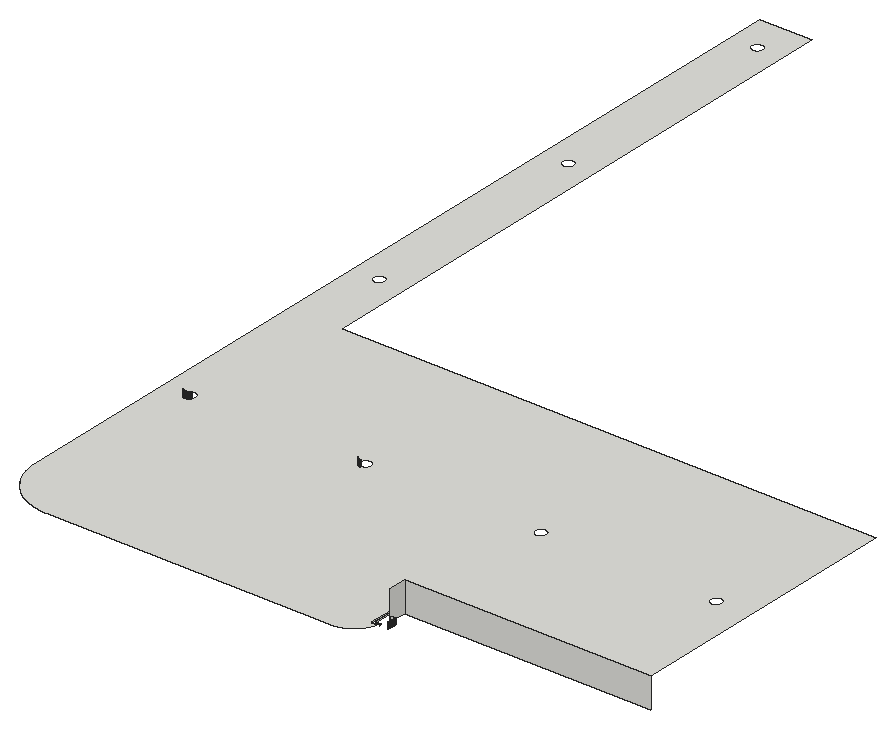
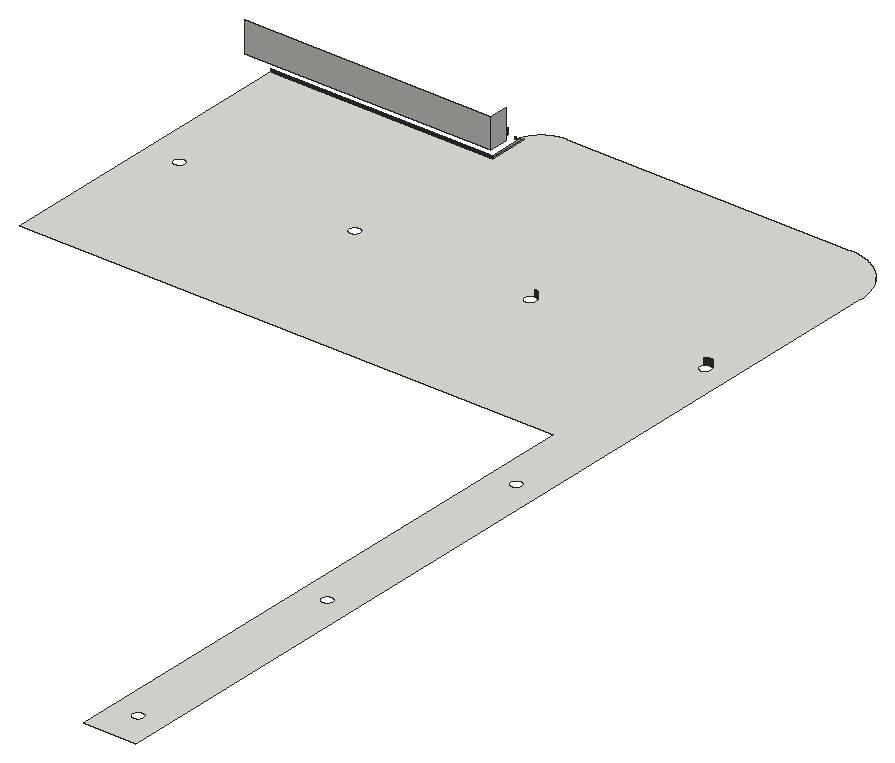
# SketchUp Ruby script. Lengths in inches.
U = 1.inch
M = Sketchup.active_model
def pt(a) = Geom::Point3d.new(a.map { |v| v * U })
def face(e, loops, mat)
  f = e.add_face(loops[0].map { |a| pt(a) })
  loops[1..].each { |l| e.add_face(l.map { |a| pt(a) }).erase! }
  f.material = f.back_material = mat if mat
  f
end
# faces: each face lists its corners as indices into pts; further lists are holes
def faces(e, pts, list, mat = nil) = list.each { |f| face(e, (f[0].is_a?(Array) ? f : [f]).map { |l| l.map { |i| pts[i] } }, mat) }
# xy, xz, yz: faces in a plane at the given z, y or x. An outline is a flat list of corners, or four numbers for a rectangle; further outlines are holes
def ring(l) = l.size == 4 ? [[l[0], l[1]], [l[2], l[1]], [l[2], l[3]], [l[0], l[3]]] : l.each_slice(2).to_a
def flat(e, list, mat, &to3) = list.each { |f| face(e, (f[0].is_a?(Array) ? f : [f]).map { |l| ring(l).map { |u, v| to3.(u, v) } }, mat) }
def xy(e, z, list, mat = nil) = flat(e, list, mat) { |x, y| [x, y, z] }
def xz(e, y, list, mat = nil) = flat(e, list, mat) { |x, z| [x, y, z] }
def yz(e, x, list, mat = nil) = flat(e, list, mat) { |y, z| [x, y, z] }
def lines(e, pts, list) = list.each { |a, b| e.add_line(pt(pts[a]), pt(pts[b])) }
# prism: a flat outline (further loops are holes) pulled along v
def prism(e, loops, v, mat = nil)
  f = face(e, loops, mat); d = Geom::Vector3d.new(v.map { |x| x * U })
  f.pushpull(f.normal.samedirection?(d) ? d.length : -d.length)
end
def box(e, o, s, mat = nil) = prism(e, [[o, [o[0] + s[0], o[1], o[2]], [o[0] + s[0], o[1] + s[1], o[2]], [o[0], o[1] + s[1], o[2]]]], [0, 0, s[2]], mat)
def at(x, y, z, deg = 0) = Geom::Transformation.translation(pt([x, y, z])) * Geom::Transformation.rotation(ORIGIN, Z_AXIS, deg.degrees)
def axes(o, x, y, z) = Geom::Transformation.new([*x, 0, *y, 0, *z, 0, *pt(o).to_a, 1])
def part(name) = M.definitions.add(name)
# library, detail: a bought-in or finely detailed component or shape, given as its bounding box
def library(name, o, s) = part(name).tap { |d| box(d.entities, o, s) }
def detail(e, o, s) = box(e.add_group.entities, o, s)
def put(e, d, t, mat = nil) = e.add_instance(d, t).tap { |i| i.material = mat if mat }
def group(e, t, mat = nil) = e.add_group.tap { |g| g.transformation = t; g.material = mat if mat }.entities
root = M.entities
M.materials.add("1496 AP 8293 CARBON COPY").color = [58, 58, 58]
xy(root,258,[[[43.63,69,43.27,69.01,42.9,69.02,42.53,69.04,42.17,69.06,41.8,69.09,41.4375,69.12,41.07,69.15,40.71,69.19,40.35,69.24,39.98,69.29,39.62,69.34,39.26,69.4,38.18,69.61,37.46,69.77,37.11,69.86,36.75,69.95,36.05,70.15,35.35,70.37,34.65,70.61,34.31,70.73,33.97,70.86,33.625,70.99,33.28,71.13,32.95,71.27,32.61,71.42,32.28,71.57,31.29,72.05,30.96,72.22,30.64,72.39,30,72.75,29.68,72.9375,29.37,73.125,29.06,73.32,28.44,73.72,28.14,73.92,27.84,74.13,27.54,74.35,27.25,74.56,26.95,74.79,26.67,75.01,26.38,75.24,26.1,75.47,25.26,76.19,24.99,76.4375,24.73,76.69,24.46,76.94,23.94,77.46,23.69,77.73,23.4375,77.99,23.19,78.26,22.47,79.1,22.24,79.38,22.01,79.67,21.79,79.95,21.56,80.25,21.35,80.54,21.13,80.84,20.92,81.14,20.72,81.44,20.32,82.06,20.125,82.37,19.9375,82.68,19.75,83,19.39,83.64,19.22,83.96,19.05,84.29,18.57,85.28,18.42,85.61,18.27,85.95,18.13,86.28,17.99,86.625,17.86,86.97,17.73,87.31,17.61,87.65,17.37,88.35,17.15,89.05,16.95,89.75,16.86,90.11,16.77,90.46,16.61,91.18,16.4,92.26,16.34,92.62,16.29,92.98,16.24,93.35,16.19,93.71,16.15,94.07,16.12,94.4375,16.09,94.8,16.06,95.17,16.04,95.53,16.02,95.9,16.01,96.27,16,96.63,16,550,42,550,42,256,309,256,309,99,198,99,198,80,200.2,80,200.15,79.86,200.01,79.46,199.9375,79.27,199.86,79.07,199.78,78.88,199.7,78.68,199.62,78.49,199.35,77.92,199.26,77.74,199.16,77.55,199.0625,77.37,198.96,77.18,198.86,77,198.53,76.46,198.42,76.29,198.3,76.11,198.1875,75.9375,198.07,75.77,197.94,75.6,197.82,75.43,197.56,75.09,197.17,74.61,196.89,74.29,196.61,73.99,196.46,73.84,196.3125,73.6875,196.16,73.54,196.01,73.39,195.71,73.11,195.39,72.83,194.91,72.44,194.57,72.18,194.4,72.06,194.23,71.93,194.0625,71.8125,193.89,71.7,193.71,71.58,193.54,71.47,193,71.14,192.82,71.04,192.63,70.9375,192.45,70.84,192.26,70.74,192.08,70.65,191.51,70.38,191.32,70.3,191.12,70.22,190.93,70.14,190.73,70.0625,190.54,69.99,189.94,69.78,189.34,69.6,189.14,69.55,188.9375,69.49,188.74,69.44,188.53,69.39,188.33,69.35,188.12,69.31,187.92,69.27,187.71,69.23,187.5,69.2,187.3,69.17,186.88,69.11,186.46,69.07,186.26,69.05,186.05,69.03,185.63,69.01,185.42,69.01,185.21,69],[28.92,410.83,29.08,410.83,29.16,410.84,29.24,410.84,29.3125,410.85,29.39,410.86,29.55,410.88,29.7,410.92,29.78,410.9375,29.85,410.96,29.93,410.98,30,411.01,30.08,411.03,30.15,411.0625,30.22,411.09,30.36,411.16,30.57,411.28,30.63,411.32,30.7,411.36,30.76,411.41,30.83,411.45,31.01,411.6,31.18,411.77,31.23,411.83,31.28,411.88,31.33,411.95,31.43,412.07,31.47,412.13,31.52,412.2,31.56,412.27,31.6,412.33,31.64,412.4,31.67,412.47,31.71,412.54,31.74,412.61,31.77,412.69,31.83,412.83,31.85,412.91,31.875,412.98,31.9,413.06,31.92,413.13,31.93,413.21,31.95,413.29,31.96,413.36,32,413.68,32,413.99,31.98,414.15,31.97,414.22,31.95,414.38,31.93,414.46,31.92,414.53,31.9,414.61,31.875,414.69,31.85,414.76,31.83,414.83,31.8,414.91,31.74,415.05,31.71,415.125,31.67,415.2,31.64,415.26,31.52,415.47,31.47,415.53,31.43,415.6,31.18,415.9,31.12,415.95,31.07,416.01,31.01,416.0625,30.95,416.11,30.83,416.21,30.76,416.26,30.7,416.31,30.63,416.35,30.57,416.39,30.36,416.51,30.08,416.63,30,416.66,29.93,416.6875,29.85,416.71,29.78,416.73,29.7,416.75,29.625,416.77,29.55,416.78,29.47,416.8,29.39,416.81,29.3125,416.82,29.24,416.82,29.16,416.83,28.84,416.83,28.76,416.82,28.6875,416.82,28.61,416.81,28.53,416.8,28.45,416.78,28.375,416.77,28.3,416.75,28.22,416.73,28.15,416.71,28.07,416.6875,28,416.66,27.92,416.63,27.64,416.51,27.43,416.39,27.37,416.35,27.3,416.31,27.24,416.26,27.17,416.21,27.05,416.11,26.99,416.0625,26.93,416.01,26.88,415.95,26.82,415.9,26.57,415.6,26.53,415.53,26.48,415.47,26.36,415.26,26.33,415.2,26.29,415.125,26.26,415.05,26.2,414.91,26.17,414.83,26.15,414.76,26.125,414.69,26.1,414.61,26.08,414.53,26.07,414.46,26.05,414.38,26.03,414.22,26.02,414.15,26,413.99,26,413.68,26.04,413.36,26.05,413.29,26.07,413.21,26.08,413.13,26.1,413.06,26.125,412.98,26.15,412.91,26.17,412.83,26.23,412.69,26.26,412.61,26.29,412.54,26.33,412.47,26.36,412.4,26.4,412.33,26.44,412.27,26.48,412.2,26.53,412.13,26.57,412.07,26.67,411.95,26.72,411.88,26.77,411.83,26.82,411.77,26.99,411.6,27.17,411.45,27.24,411.41,27.3,411.36,27.37,411.32,27.43,411.28,27.64,411.16,27.78,411.09,27.85,411.0625,27.92,411.03,28,411.01,28.07,410.98,28.15,410.96,28.22,410.9375,28.3,410.92,28.45,410.88,28.61,410.86,28.6875,410.85,28.76,410.84,28.84,410.84],[28.84,292.67,29.16,292.67,29.24,292.68,29.3125,292.68,29.39,292.69,29.47,292.7,29.55,292.72,29.625,292.73,29.7,292.75,29.78,292.77,29.85,292.79,29.93,292.8125,30,292.84,30.08,292.87,30.36,292.99,30.57,293.11,30.63,293.15,30.7,293.19,30.76,293.24,30.83,293.29,30.95,293.39,31.01,293.4375,31.07,293.49,31.12,293.55,31.18,293.6,31.43,293.9,31.47,293.97,31.52,294.03,31.64,294.24,31.67,294.3,31.71,294.375,31.74,294.45,31.8,294.59,31.83,294.67,31.85,294.74,31.875,294.81,31.9,294.89,31.92,294.97,31.93,295.04,31.95,295.12,31.97,295.28,31.98,295.35,32,295.51,32,295.82,31.96,296.14,31.95,296.21,31.93,296.29,31.92,296.37,31.9,296.44,31.875,296.52,31.85,296.59,31.83,296.67,31.77,296.81,31.74,296.89,31.71,296.96,31.67,297.03,31.64,297.1,31.6,297.17,31.56,297.23,31.52,297.3,31.47,297.37,31.43,297.43,31.33,297.55,31.28,297.62,31.23,297.67,31.18,297.73,31.01,297.9,30.83,298.05,30.76,298.09,30.7,298.14,30.63,298.18,30.57,298.22,30.36,298.34,30.22,298.41,30.15,298.4375,30.08,298.47,30,298.49,29.93,298.52,29.85,298.54,29.78,298.5625,29.7,298.58,29.55,298.62,29.39,298.64,29.3125,298.65,29.24,298.66,29.16,298.66,29.08,298.67,28.92,298.67,28.84,298.66,28.76,298.66,28.6875,298.65,28.61,298.64,28.45,298.62,28.3,298.58,28.22,298.5625,28.15,298.54,28.07,298.52,28,298.49,27.92,298.47,27.85,298.4375,27.78,298.41,27.64,298.34,27.43,298.22,27.37,298.18,27.3,298.14,27.24,298.09,27.17,298.05,26.99,297.9,26.82,297.73,26.77,297.67,26.72,297.62,26.67,297.55,26.57,297.43,26.53,297.37,26.48,297.3,26.44,297.23,26.4,297.17,26.36,297.1,26.33,297.03,26.29,296.96,26.26,296.89,26.23,296.81,26.17,296.67,26.15,296.59,26.125,296.52,26.1,296.44,26.08,296.37,26.07,296.29,26.05,296.21,26.04,296.14,26,295.82,26,295.51,26.02,295.35,26.03,295.28,26.05,295.12,26.07,295.04,26.08,294.97,26.1,294.89,26.125,294.81,26.15,294.74,26.17,294.67,26.2,294.59,26.26,294.45,26.29,294.375,26.33,294.3,26.36,294.24,26.48,294.03,26.53,293.97,26.57,293.9,26.82,293.6,26.88,293.55,26.93,293.49,26.99,293.4375,27.05,293.39,27.17,293.29,27.24,293.24,27.3,293.19,27.37,293.15,27.43,293.11,27.64,292.99,27.92,292.87,28,292.84,28.07,292.8125,28.15,292.79,28.22,292.77,28.3,292.75,28.375,292.73,28.45,292.72,28.53,292.7,28.61,292.69,28.6875,292.68,28.76,292.68],[28.84,174.5,29.16,174.5,29.24,174.51,29.3125,174.52,29.39,174.53,29.55,174.55,29.625,174.57,29.7,174.58,29.78,174.6,29.85,174.625,29.93,174.65,30,174.67,30.08,174.7,30.29,174.79,30.36,174.83,30.43,174.86,30.57,174.94,30.63,174.98,30.7,175.03,30.76,175.07,30.83,175.12,31.07,175.32,31.12,175.38,31.18,175.43,31.38,175.67,31.43,175.74,31.47,175.8,31.52,175.87,31.56,175.93,31.64,176.07,31.67,176.14,31.71,176.21,31.8,176.42,31.83,176.5,31.85,176.57,31.875,176.65,31.9,176.72,31.92,176.8,31.93,176.875,31.95,176.95,31.97,177.11,31.98,177.1875,31.99,177.26,32,177.34,32,177.66,31.99,177.74,31.98,177.8125,31.97,177.89,31.95,178.05,31.93,178.125,31.92,178.2,31.9,178.28,31.875,178.35,31.85,178.43,31.83,178.5,31.8,178.58,31.71,178.79,31.67,178.86,31.64,178.93,31.56,179.07,31.52,179.13,31.47,179.2,31.43,179.26,31.38,179.33,31.18,179.57,31.12,179.62,31.07,179.68,30.83,179.88,30.76,179.93,30.7,179.97,30.63,180.02,30.57,180.06,30.43,180.14,30.36,180.17,30.29,180.21,30.08,180.3,30,180.33,29.93,180.35,29.85,180.375,29.78,180.4,29.7,180.42,29.625,180.43,29.55,180.45,29.39,180.47,29.3125,180.48,29.24,180.49,29.16,180.5,28.84,180.5,28.76,180.49,28.6875,180.48,28.61,180.47,28.45,180.45,28.375,180.43,28.3,180.42,28.22,180.4,28.15,180.375,28.07,180.35,28,180.33,27.92,180.3,27.71,180.21,27.64,180.17,27.57,180.14,27.43,180.06,27.37,180.02,27.3,179.97,27.24,179.93,27.17,179.88,26.93,179.68,26.88,179.62,26.82,179.57,26.62,179.33,26.57,179.26,26.53,179.2,26.48,179.13,26.44,179.07,26.36,178.93,26.33,178.86,26.29,178.79,26.2,178.58,26.17,178.5,26.15,178.43,26.125,178.35,26.1,178.28,26.08,178.2,26.07,178.125,26.05,178.05,26.03,177.89,26.02,177.8125,26.01,177.74,26,177.66,26,177.34,26.01,177.26,26.02,177.1875,26.03,177.11,26.05,176.95,26.07,176.875,26.08,176.8,26.1,176.72,26.125,176.65,26.15,176.57,26.17,176.5,26.2,176.42,26.29,176.21,26.33,176.14,26.36,176.07,26.44,175.93,26.48,175.87,26.53,175.8,26.57,175.74,26.62,175.67,26.82,175.43,26.88,175.38,26.93,175.32,27.17,175.12,27.24,175.07,27.3,175.03,27.37,174.98,27.43,174.94,27.57,174.86,27.64,174.83,27.71,174.79,27.92,174.7,28,174.67,28.07,174.65,28.15,174.625,28.22,174.6,28.3,174.58,28.375,174.57,28.45,174.55,28.61,174.53,28.6875,174.52,28.76,174.51],[28.84,529,29.16,529,29.24,529.01,29.3125,529.02,29.39,529.03,29.55,529.05,29.625,529.07,29.7,529.08,29.78,529.1,29.85,529.125,29.93,529.15,30,529.17,30.08,529.2,30.29,529.29,30.36,529.33,30.43,529.36,30.57,529.44,30.63,529.48,30.7,529.53,30.76,529.57,30.83,529.62,31.07,529.82,31.12,529.88,31.18,529.93,31.38,530.17,31.43,530.24,31.47,530.3,31.52,530.37,31.56,530.43,31.64,530.57,31.67,530.64,31.71,530.71,31.8,530.92,31.83,531,31.85,531.07,31.875,531.15,31.9,531.22,31.92,531.3,31.93,531.375,31.95,531.45,31.97,531.61,31.98,531.6875,31.99,531.76,32,531.84,32,532.16,31.99,532.24,31.98,532.3125,31.97,532.39,31.95,532.55,31.93,532.625,31.92,532.7,31.9,532.78,31.875,532.85,31.85,532.93,31.83,533,31.8,533.08,31.71,533.29,31.67,533.36,31.64,533.43,31.56,533.57,31.52,533.63,31.47,533.7,31.43,533.76,31.38,533.83,31.18,534.07,31.12,534.12,31.07,534.18,30.83,534.38,30.76,534.43,30.7,534.47,30.63,534.52,30.57,534.56,30.43,534.64,30.36,534.67,30.29,534.71,30.08,534.8,30,534.83,29.93,534.85,29.85,534.875,29.78,534.9,29.7,534.92,29.625,534.93,29.55,534.95,29.39,534.97,29.3125,534.98,29.24,534.99,29.16,535,28.84,535,28.76,534.99,28.6875,534.98,28.61,534.97,28.45,534.95,28.375,534.93,28.3,534.92,28.22,534.9,28.15,534.875,28.07,534.85,28,534.83,27.92,534.8,27.71,534.71,27.64,534.67,27.57,534.64,27.43,534.56,27.37,534.52,27.3,534.47,27.24,534.43,27.17,534.38,26.93,534.18,26.88,534.12,26.82,534.07,26.62,533.83,26.57,533.76,26.53,533.7,26.48,533.63,26.44,533.57,26.36,533.43,26.33,533.36,26.29,533.29,26.2,533.08,26.17,533,26.15,532.93,26.125,532.85,26.1,532.78,26.08,532.7,26.07,532.625,26.05,532.55,26.03,532.39,26.02,532.3125,26.01,532.24,26,532.16,26,531.84,26.01,531.76,26.02,531.6875,26.03,531.61,26.05,531.45,26.07,531.375,26.08,531.3,26.1,531.22,26.125,531.15,26.15,531.07,26.17,531,26.2,530.92,26.29,530.71,26.33,530.64,26.36,530.57,26.44,530.43,26.48,530.37,26.53,530.3,26.57,530.24,26.62,530.17,26.82,529.93,26.88,529.88,26.93,529.82,27.17,529.62,27.24,529.57,27.3,529.53,27.37,529.48,27.43,529.44,27.57,529.36,27.64,529.33,27.71,529.29,27.92,529.2,28,529.17,28.07,529.15,28.15,529.125,28.22,529.1,28.3,529.08,28.375,529.07,28.45,529.05,28.61,529.03,28.6875,529.02,28.76,529.01],[116.51,174.5,116.82,174.5,117.14,174.54,117.21,174.55,117.29,174.57,117.37,174.58,117.44,174.6,117.52,174.625,117.59,174.65,117.67,174.67,117.81,174.73,117.89,174.76,117.96,174.79,118.03,174.83,118.1,174.86,118.17,174.9,118.23,174.94,118.3,174.98,118.37,175.03,118.43,175.07,118.55,175.17,118.62,175.22,118.67,175.27,118.73,175.32,118.9,175.49,119.05,175.67,119.09,175.74,119.14,175.8,119.18,175.87,119.22,175.93,119.34,176.14,119.41,176.28,119.4375,176.35,119.47,176.42,119.49,176.5,119.52,176.57,119.54,176.65,119.5625,176.72,119.58,176.8,119.62,176.95,119.64,177.11,119.65,177.1875,119.66,177.26,119.66,177.34,119.67,177.42,119.67,177.58,119.66,177.66,119.66,177.74,119.65,177.8125,119.64,177.89,119.62,178.05,119.58,178.2,119.5625,178.28,119.54,178.35,119.52,178.43,119.49,178.5,119.47,178.58,119.4375,178.65,119.41,178.72,119.34,178.86,119.22,179.07,119.18,179.13,119.14,179.2,119.09,179.26,119.05,179.33,118.9,179.51,118.73,179.68,118.67,179.73,118.62,179.78,118.55,179.83,118.43,179.93,118.37,179.97,118.3,180.02,118.23,180.06,118.17,180.1,118.1,180.14,118.03,180.17,117.96,180.21,117.89,180.24,117.81,180.27,117.67,180.33,117.59,180.35,117.52,180.375,117.44,180.4,117.37,180.42,117.29,180.43,117.21,180.45,117.14,180.46,116.82,180.5,116.51,180.5,116.35,180.48,116.28,180.47,116.12,180.45,116.04,180.43,115.97,180.42,115.89,180.4,115.81,180.375,115.74,180.35,115.67,180.33,115.59,180.3,115.45,180.24,115.375,180.21,115.3,180.17,115.24,180.14,115.03,180.02,114.97,179.97,114.9,179.93,114.6,179.68,114.55,179.62,114.49,179.57,114.4375,179.51,114.39,179.45,114.29,179.33,114.24,179.26,114.19,179.2,114.15,179.13,114.11,179.07,113.99,178.86,113.87,178.58,113.84,178.5,113.8125,178.43,113.79,178.35,113.77,178.28,113.75,178.2,113.73,178.125,113.72,178.05,113.7,177.97,113.69,177.89,113.68,177.8125,113.68,177.74,113.67,177.66,113.67,177.34,113.68,177.26,113.68,177.1875,113.69,177.11,113.7,177.03,113.72,176.95,113.73,176.875,113.75,176.8,113.77,176.72,113.79,176.65,113.8125,176.57,113.84,176.5,113.87,176.42,113.99,176.14,114.11,175.93,114.15,175.87,114.19,175.8,114.24,175.74,114.29,175.67,114.39,175.55,114.4375,175.49,114.49,175.43,114.55,175.38,114.6,175.32,114.9,175.07,114.97,175.03,115.03,174.98,115.24,174.86,115.3,174.83,115.375,174.79,115.45,174.76,115.59,174.7,115.67,174.67,115.74,174.65,115.81,174.625,115.89,174.6,115.97,174.58,116.04,174.57,116.12,174.55,116.28,174.53,116.35,174.52],[204.18,174.5,204.49,174.5,204.65,174.52,204.72,174.53,204.88,174.55,204.96,174.57,205.03,174.58,205.11,174.6,205.19,174.625,205.26,174.65,205.33,174.67,205.41,174.7,205.55,174.76,205.625,174.79,205.7,174.83,205.76,174.86,205.97,174.98,206.03,175.03,206.1,175.07,206.4,175.32,206.45,175.38,206.51,175.43,206.5625,175.49,206.61,175.55,206.71,175.67,206.76,175.74,206.81,175.8,206.85,175.87,206.89,175.93,207.01,176.14,207.13,176.42,207.16,176.5,207.1875,176.57,207.21,176.65,207.23,176.72,207.25,176.8,207.27,176.875,207.28,176.95,207.3,177.03,207.31,177.11,207.32,177.1875,207.32,177.26,207.33,177.34,207.33,177.66,207.32,177.74,207.32,177.8125,207.31,177.89,207.3,177.97,207.28,178.05,207.27,178.125,207.25,178.2,207.23,178.28,207.21,178.35,207.1875,178.43,207.16,178.5,207.13,178.58,207.01,178.86,206.89,179.07,206.85,179.13,206.81,179.2,206.76,179.26,206.71,179.33,206.61,179.45,206.5625,179.51,206.51,179.57,206.45,179.62,206.4,179.68,206.1,179.93,206.03,179.97,205.97,180.02,205.76,180.14,205.7,180.17,205.625,180.21,205.55,180.24,205.41,180.3,205.33,180.33,205.26,180.35,205.19,180.375,205.11,180.4,205.03,180.42,204.96,180.43,204.88,180.45,204.72,180.47,204.65,180.48,204.49,180.5,204.18,180.5,203.86,180.46,203.79,180.45,203.71,180.43,203.63,180.42,203.56,180.4,203.48,180.375,203.41,180.35,203.33,180.33,203.19,180.27,203.11,180.24,203.04,180.21,202.97,180.17,202.9,180.14,202.83,180.1,202.77,180.06,202.7,180.02,202.63,179.97,202.57,179.93,202.45,179.83,202.38,179.78,202.33,179.73,202.27,179.68,202.1,179.51,201.95,179.33,201.91,179.26,201.86,179.2,201.82,179.13,201.78,179.07,201.66,178.86,201.59,178.72,201.5625,178.65,201.53,178.58,201.51,178.5,201.48,178.43,201.46,178.35,201.4375,178.28,201.42,178.2,201.38,178.05,201.36,177.89,201.35,177.8125,201.34,177.74,201.34,177.66,201.33,177.58,201.33,177.42,201.34,177.34,201.34,177.26,201.35,177.1875,201.36,177.11,201.38,176.95,201.42,176.8,201.4375,176.72,201.46,176.65,201.48,176.57,201.51,176.5,201.53,176.42,201.5625,176.35,201.59,176.28,201.66,176.14,201.78,175.93,201.82,175.87,201.86,175.8,201.91,175.74,201.95,175.67,202.1,175.49,202.27,175.32,202.33,175.27,202.38,175.22,202.45,175.17,202.57,175.07,202.63,175.03,202.7,174.98,202.77,174.94,202.83,174.9,202.9,174.86,202.97,174.83,203.04,174.79,203.11,174.76,203.19,174.73,203.33,174.67,203.41,174.65,203.48,174.625,203.56,174.6,203.63,174.58,203.71,174.57,203.79,174.55,203.86,174.54],[291.84,174.5,292.16,174.5,292.24,174.51,292.3125,174.52,292.39,174.53,292.55,174.55,292.625,174.57,292.7,174.58,292.78,174.6,292.85,174.625,292.93,174.65,293,174.67,293.08,174.7,293.29,174.79,293.36,174.83,293.43,174.86,293.57,174.94,293.63,174.98,293.7,175.03,293.76,175.07,293.83,175.12,294.07,175.32,294.12,175.38,294.18,175.43,294.38,175.67,294.43,175.74,294.47,175.8,294.52,175.87,294.56,175.93,294.64,176.07,294.67,176.14,294.71,176.21,294.8,176.42,294.83,176.5,294.85,176.57,294.875,176.65,294.9,176.72,294.92,176.8,294.93,176.875,294.95,176.95,294.97,177.11,294.98,177.1875,294.99,177.26,295,177.34,295,177.66,294.99,177.74,294.98,177.8125,294.97,177.89,294.95,178.05,294.93,178.125,294.92,178.2,294.9,178.28,294.875,178.35,294.85,178.43,294.83,178.5,294.8,178.58,294.71,178.79,294.67,178.86,294.64,178.93,294.56,179.07,294.52,179.13,294.47,179.2,294.43,179.26,294.38,179.33,294.18,179.57,294.12,179.62,294.07,179.68,293.83,179.88,293.76,179.93,293.7,179.97,293.63,180.02,293.57,180.06,293.43,180.14,293.36,180.17,293.29,180.21,293.08,180.3,293,180.33,292.93,180.35,292.85,180.375,292.78,180.4,292.7,180.42,292.625,180.43,292.55,180.45,292.39,180.47,292.3125,180.48,292.24,180.49,292.16,180.5,291.84,180.5,291.76,180.49,291.6875,180.48,291.61,180.47,291.45,180.45,291.375,180.43,291.3,180.42,291.22,180.4,291.15,180.375,291.07,180.35,291,180.33,290.92,180.3,290.71,180.21,290.64,180.17,290.57,180.14,290.43,180.06,290.37,180.02,290.3,179.97,290.24,179.93,290.17,179.88,289.93,179.68,289.88,179.62,289.82,179.57,289.62,179.33,289.57,179.26,289.53,179.2,289.48,179.13,289.44,179.07,289.36,178.93,289.33,178.86,289.29,178.79,289.2,178.58,289.17,178.5,289.15,178.43,289.125,178.35,289.1,178.28,289.08,178.2,289.07,178.125,289.05,178.05,289.03,177.89,289.02,177.8125,289.01,177.74,289,177.66,289,177.34,289.01,177.26,289.02,177.1875,289.03,177.11,289.05,176.95,289.07,176.875,289.08,176.8,289.1,176.72,289.125,176.65,289.15,176.57,289.17,176.5,289.2,176.42,289.29,176.21,289.33,176.14,289.36,176.07,289.44,175.93,289.48,175.87,289.53,175.8,289.57,175.74,289.62,175.67,289.82,175.43,289.88,175.38,289.93,175.32,290.17,175.12,290.24,175.07,290.3,175.03,290.37,174.98,290.43,174.94,290.57,174.86,290.64,174.83,290.71,174.79,290.92,174.7,291,174.67,291.07,174.65,291.15,174.625,291.22,174.6,291.3,174.58,291.375,174.57,291.45,174.55,291.61,174.53,291.6875,174.52,291.76,174.51]]])
xz(root,81,[[199,258,201.52,258.5]])
xz(root,85,[[203,258,206,261]])
xz(root,94,[[203,258,326,273]])
xz(root,98,[[199,258,310,258.5]])
xz(root,99,[[198,258,309,258.5]])
xz(root,174.5,[[28.84,258,28.92,261],[28.92,258,29,261],[29,258,29.08,261],[29.08,258,29.16,261],[116.51,258,116.59,261],
  [116.59,258,116.67,261]])
yz(root,198,[[80,258,99,258.5]])
yz(root,199,[[81,258,98,258.5]])
yz(root,203,[[85,258,94,273]])
yz(root,206,[[84.73,258,85,261]],"1496 AP 8293 CARBON COPY")
p = [[201.42,80.6,258],[201.36,80.39,258],[201.36,80.39,258.5],[201.42,80.6,258.5],[205.54,80.63,261],[205.48,80.37,261],
  [205.48,80.37,258],[205.54,80.63,258],[21.13,80.84,258],[21.35,80.54,258],[21.35,80.54,258.5],[21.13,80.84,258.5],
  [201.48,80.82,258],[201.48,80.82,258.5],[205.6,80.9,261],[205.6,80.9,258],[20.92,81.14,258],[20.92,81.14,258.5],
  [201.52,81,258],[201.52,81,258.5],[205.65,81.17,261],[205.65,81.17,258],[20.72,81.44,258],[20.72,81.44,258.5],
  [205.7,81.44,261],[205.7,81.44,258],[205.74,81.71,261],[205.74,81.71,258],[205.78,81.99,261],[205.78,81.99,258],
  [205.82,82.26,261],[205.82,82.26,258],[205.85,82.53,261],[205.85,82.53,258],[205.88,82.8,261],[205.88,82.8,258],
  [205.91,83.08,261],[205.91,83.08,258],[205.94,83.35,261],[205.94,83.35,258],[205.96,83.625,261],[205.96,83.625,258],
  [205.97,83.9,261],[205.97,83.9,258],[205.98,84.18,261],[205.98,84.18,258],[205.99,84.45,261],[205.99,84.45,258],
  [206,84.73,261],[206,84.73,258],[28.53,174.54,258],[28.45,174.55,258],[28.45,174.55,261],[28.53,174.54,261],
  [28.61,174.53,258],[28.61,174.53,261],[28.6875,174.52,258],[28.6875,174.52,261],[28.76,174.51,258],[28.76,174.51,261],
  [28.84,174.5,258],[28.84,174.5,261],[29.24,174.51,258],[29.16,174.5,258],[29.16,174.5,261],[29.24,174.51,261],
  [29.3125,174.52,258],[29.3125,174.52,261],[29.39,174.53,258],[29.39,174.53,261],[29.47,174.54,258],[29.47,174.54,261],
  [29.55,174.55,258],[29.55,174.55,261],[116.2,174.54,258],[116.12,174.55,258],[116.12,174.55,261],[116.2,174.54,261],
  [116.28,174.53,258],[116.28,174.53,261],[116.35,174.52,258],[116.35,174.52,261],[116.43,174.51,258],[116.43,174.51,261],
  [116.51,174.5,258],[116.51,174.5,261],[28.07,174.65,258],[28,174.67,258],[28,174.67,261],[28.07,174.65,261],
  [28.15,174.625,258],[28.15,174.625,261],[28.22,174.6,258],[28.22,174.6,261],[28.3,174.58,258],[28.3,174.58,261],
  [28.375,174.57,258],[28.375,174.57,261],[29.625,174.57,258],[29.625,174.57,261],[29.7,174.58,258],[29.7,174.58,261],
  [29.78,174.6,258],[29.78,174.6,261],[29.85,174.625,258],[29.85,174.625,261],[29.93,174.65,258],[29.93,174.65,261],
  [30,174.67,258],[30,174.67,261],[115.74,174.65,258],[115.67,174.67,258],[115.67,174.67,261],[115.74,174.65,261],
  [115.81,174.625,258],[115.81,174.625,261],[115.89,174.6,258],[115.89,174.6,261],[115.97,174.58,258],[115.97,174.58,261],
  [116.04,174.57,258],[116.04,174.57,261],[27.85,174.73,258],[27.78,174.76,258],[27.78,174.76,261],[27.85,174.73,261],
  [27.92,174.7,258],[27.92,174.7,261],[30.08,174.7,258],[30.08,174.7,261],[30.15,174.73,258],[30.15,174.73,261],
  [30.22,174.76,258],[30.22,174.76,261],[115.52,174.73,258],[115.45,174.76,258],[115.45,174.76,261],[115.52,174.73,261],
  [115.59,174.7,258],[115.59,174.7,261],[27.64,174.83,258],[27.57,174.86,258],[27.57,174.86,261],[27.64,174.83,261],
  [27.71,174.79,258],[27.71,174.79,261],[30.29,174.79,258],[30.29,174.79,261],[30.36,174.83,258],[30.36,174.83,261],
  [30.43,174.86,258],[30.43,174.86,261],[115.3,174.83,258],[115.24,174.86,258],[115.24,174.86,261],[115.3,174.83,261],
  [115.375,174.79,258],[115.375,174.79,261],[27.43,174.94,258],[27.37,174.98,258],[27.37,174.98,261],[27.43,174.94,261],
  [27.5,174.9,258],[27.5,174.9,261],[30.5,174.9,258],[30.5,174.9,261],[30.57,174.94,258],[30.57,174.94,261],
  [30.63,174.98,258],[30.63,174.98,261],[115.1,174.94,258],[115.03,174.98,258],[115.03,174.98,261],[115.1,174.94,261],
  [115.17,174.9,258],[115.17,174.9,261],[27.3,175.03,258],[27.24,175.07,258],[27.24,175.07,261],[27.3,175.03,261],
  [30.7,175.03,258],[30.7,175.03,261],[30.76,175.07,258],[30.76,175.07,261],[114.97,175.03,258],[114.9,175.07,258],
  [114.9,175.07,261],[114.97,175.03,261],[27.17,175.12,258],[27.11,175.17,258],[27.11,175.17,261],[27.17,175.12,261],
  [30.83,175.12,258],[30.83,175.12,261],[30.89,175.17,258],[30.89,175.17,261],[114.84,175.12,258],[114.78,175.17,258],
  [114.78,175.17,261],[114.84,175.12,261],[27.05,175.22,258],[26.99,175.27,258],[26.99,175.27,261],[27.05,175.22,261],
  [30.95,175.22,258],[30.95,175.22,261],[31.01,175.27,258],[31.01,175.27,261],[114.72,175.22,258],[114.66,175.27,258],
  [114.66,175.27,261],[114.72,175.22,261],[26.93,175.32,258],[26.88,175.38,258],[26.88,175.38,261],[26.93,175.32,261],
  [31.07,175.32,258],[31.07,175.32,261],[31.12,175.38,258],[31.12,175.38,261],[114.6,175.32,258],[114.55,175.38,258],
  [114.55,175.38,261],[114.6,175.32,261],[26.82,175.43,258],[26.77,175.49,258],[26.77,175.49,261],[26.82,175.43,261],
  [31.18,175.43,258],[31.18,175.43,261],[31.23,175.49,258],[31.23,175.49,261],[114.49,175.43,258],[114.4375,175.49,258],
  [114.4375,175.49,261],[114.49,175.43,261],[26.72,175.55,258],[26.72,175.55,261],[31.28,175.55,258],[31.28,175.55,261],
  [114.39,175.55,258],[114.39,175.55,261],[26.67,175.61,258],[26.67,175.61,261],[323,94,261],[323,94,258]]
faces(root,p,[[0,1,2,3],[8,9,10,11],[12,0,3,13],[16,8,11,17],[18,12,13,19],[22,16,17,23],[50,51,52,53],[54,50,53,55],
  [56,54,55,57],[58,56,57,59],[60,58,59,61],[62,63,64,65],[66,62,65,67],[68,66,67,69],[70,68,69,71],[72,70,71,73],
  [74,75,76,77],[78,74,77,79],[80,78,79,81],[82,80,81,83],[84,82,83,85],[86,87,88,89],[90,86,89,91],[92,90,91,93],
  [94,92,93,95],[96,94,95,97],[51,96,97,52],[98,72,73,99],[100,98,99,101],[102,100,101,103],[104,102,103,105],[106,104,105,107],
  [108,106,107,109],[110,111,112,113],[114,110,113,115],[116,114,115,117],[118,116,117,119],[120,118,119,121],[75,120,121,76],[122,123,124,125],
  [126,122,125,127],[87,126,127,88],[128,108,109,129],[130,128,129,131],[132,130,131,133],[134,135,136,137],[138,134,137,139],[111,138,139,112],
  [140,141,142,143],[144,140,143,145],[123,144,145,124],[146,132,133,147],[148,146,147,149],[150,148,149,151],[152,153,154,155],[156,152,155,157],
  [135,156,157,136],[158,159,160,161],[162,158,161,163],[141,162,163,142],[164,150,151,165],[166,164,165,167],[168,166,167,169],[170,171,172,173],
  [174,170,173,175],[153,174,175,154],[176,177,178,179],[159,176,179,160],[180,168,169,181],[182,180,181,183],[184,185,186,187],[171,184,187,172],
  [188,189,190,191],[177,188,191,178],[192,182,183,193],[194,192,193,195],[196,197,198,199],[185,196,199,186],[200,201,202,203],[189,200,203,190],
  [204,194,195,205],[206,204,205,207],[208,209,210,211],[197,208,211,198],[212,213,214,215],[201,212,215,202],[216,206,207,217],[218,216,217,219],
  [220,221,222,223],[209,220,223,210],[224,225,226,227],[213,224,227,214],[228,218,219,229],[230,228,229,231],[232,233,234,235],[221,232,235,222],
  [225,236,237,226],[238,230,231,239],[233,240,241,234],[236,242,243,237]])
faces(root,p,[[4,5,6,7],[14,4,7,15],[20,14,15,21],[24,20,21,25],[26,24,25,27],[28,26,27,29],[30,28,29,31],[32,30,31,33],
  [34,32,33,35],[36,34,35,37],[38,36,37,39],[40,38,39,41],[42,40,41,43],[44,42,43,45],[46,44,45,47],[48,46,47,49]],"1496 AP 8293 CARBON COPY")
lines(root,p,[[244,245]])
